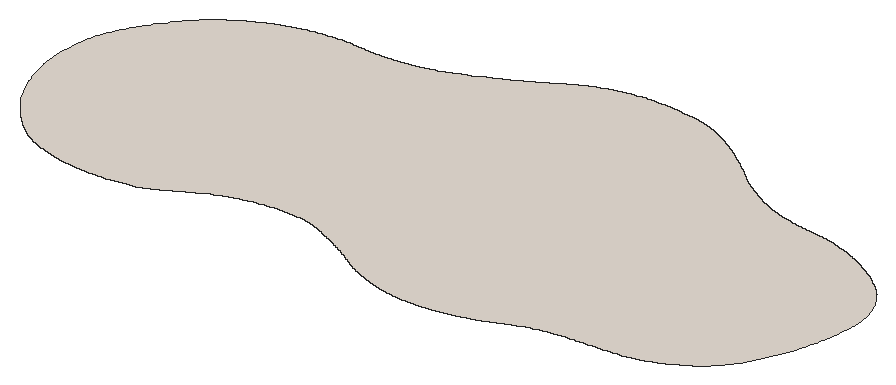
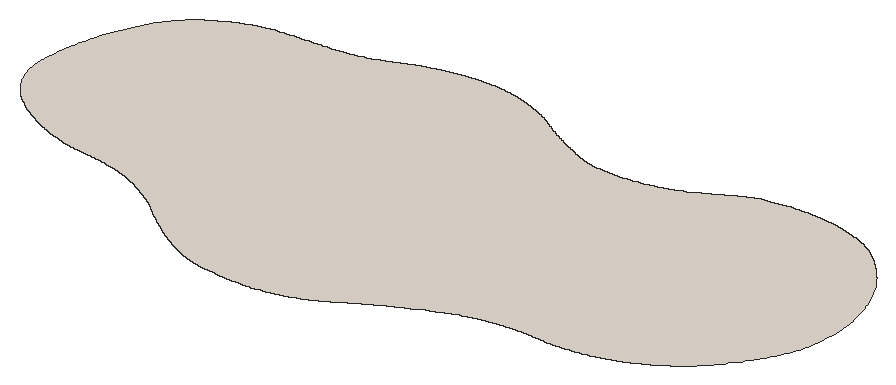
# SketchUp Ruby script. Lengths in inches.
U = 1.inch
M = Sketchup.active_model
def pt(a) = Geom::Point3d.new(a.map { |v| v * U })
def face(e, loops, mat)
  f = e.add_face(loops[0].map { |a| pt(a) })
  loops[1..].each { |l| e.add_face(l.map { |a| pt(a) }).erase! }
  f.material = f.back_material = mat if mat
  f
end
# faces: each face lists its corners as indices into pts; further lists are holes
def faces(e, pts, list, mat = nil) = list.each { |f| face(e, (f[0].is_a?(Array) ? f : [f]).map { |l| l.map { |i| pts[i] } }, mat) }
# xy, xz, yz: faces in a plane at the given z, y or x. An outline is a flat list of corners, or four numbers for a rectangle; further outlines are holes
def ring(l) = l.size == 4 ? [[l[0], l[1]], [l[2], l[1]], [l[2], l[3]], [l[0], l[3]]] : l.each_slice(2).to_a
def flat(e, list, mat, &to3) = list.each { |f| face(e, (f[0].is_a?(Array) ? f : [f]).map { |l| ring(l).map { |u, v| to3.(u, v) } }, mat) }
def xy(e, z, list, mat = nil) = flat(e, list, mat) { |x, y| [x, y, z] }
def xz(e, y, list, mat = nil) = flat(e, list, mat) { |x, z| [x, y, z] }
def yz(e, x, list, mat = nil) = flat(e, list, mat) { |y, z| [x, y, z] }
def lines(e, pts, list) = list.each { |a, b| e.add_line(pt(pts[a]), pt(pts[b])) }
# prism: a flat outline (further loops are holes) pulled along v
def prism(e, loops, v, mat = nil)
  f = face(e, loops, mat); d = Geom::Vector3d.new(v.map { |x| x * U })
  f.pushpull(f.normal.samedirection?(d) ? d.length : -d.length)
end
def box(e, o, s, mat = nil) = prism(e, [[o, [o[0] + s[0], o[1], o[2]], [o[0] + s[0], o[1] + s[1], o[2]], [o[0], o[1] + s[1], o[2]]]], [0, 0, s[2]], mat)
def at(x, y, z, deg = 0) = Geom::Transformation.translation(pt([x, y, z])) * Geom::Transformation.rotation(ORIGIN, Z_AXIS, deg.degrees)
def axes(o, x, y, z) = Geom::Transformation.new([*x, 0, *y, 0, *z, 0, *pt(o).to_a, 1])
def part(name) = M.definitions.add(name)
# library, detail: a bought-in or finely detailed component or shape, given as its bounding box
def library(name, o, s) = part(name).tap { |d| box(d.entities, o, s) }
def detail(e, o, s) = box(e.add_group.entities, o, s)
def put(e, d, t, mat = nil) = e.add_instance(d, t).tap { |i| i.material = mat if mat }
def group(e, t, mat = nil) = e.add_group.tap { |g| g.transformation = t; g.material = mat if mat }.entities
root = M.entities
M.materials.add("Marble_01_1K").color = [230, 221, 211]
xy(root,19,[[347.35,773.18,347.67,773.18,347.88,773.19,347.99,773.19,348.1,773.2,348.2,773.21,348.31,773.21,348.42,773.22,348.52,773.23,348.73,773.25,348.83,773.26,349.01,773.28,349.1,773.3,349.19,773.31,349.43,773.34,349.51,773.36,349.59,773.37,349.66,773.38,349.74,773.4,349.81,773.41,349.89,773.43,349.97,773.44,350.04,773.46,350.12,773.47,350.19,773.49,350.27,773.5,350.34,773.52,350.42,773.54,350.49,773.55,350.57,773.57,350.64,773.59,350.72,773.61,350.79,773.625,350.87,773.64,350.94,773.66,351.02,773.68,351.09,773.7,351.17,773.72,351.24,773.74,351.32,773.76,351.39,773.78,351.46,773.81,351.54,773.83,351.68,773.87,351.76,773.89,351.83,773.92,351.91,773.94,351.98,773.96,352.05,773.99,352.125,774.01,352.2,774.04,352.27,774.0625,352.34,774.09,352.42,774.11,352.49,774.14,352.5625,774.17,352.63,774.19,352.71,774.22,352.78,774.25,352.85,774.27,352.99,774.33,353.07,774.36,353.42,774.51,353.5,774.54,353.64,774.6,353.72,774.63,353.8,774.67,353.96,774.73,354.04,774.77,354.13,774.8,354.21,774.84,354.39,774.91,354.48,774.94,354.57,774.98,354.65,775.01,354.83,775.07,354.92,775.11,355.19,775.2,355.28,775.22,355.55,775.31,355.64,775.33,355.73,775.36,355.82,775.38,355.92,775.41,356.1,775.45,356.19,775.48,356.28,775.5,356.47,775.54,356.65,775.58,356.75,775.59,356.84,775.61,356.94,775.63,357.03,775.65,357.13,775.66,357.35,775.7,357.46,775.71,357.58,775.73,357.71,775.74,357.86,775.76,358.02,775.78,358.2,775.79,358.4,775.81,358.64,775.82,358.9,775.84,359.2,775.84,359.53,775.85,359.87,775.87,360.59,775.93,360.96,775.97,361.31,776.01,361.66,776.06,361.99,776.11,362.3,776.18,362.6,776.24,362.89,776.32,363.16,776.39,363.43,776.48,363.69,776.57,363.95,776.67,364.2,776.77,364.45,776.89,364.7,777,364.94,777.125,365.18,777.26,365.42,777.39,365.65,777.53,366.11,777.83,366.33,777.99,366.55,778.16,366.76,778.33,366.97,778.51,367.17,778.7,367.55,779.1,367.91,779.54,368.23,780,368.39,780.24,368.53,780.49,368.68,780.74,368.82,780.99,369.08,781.51,369.32,782.03,369.43,782.3,369.54,782.5625,369.65,782.83,369.75,783.1,369.93,783.65,370.01,783.93,370.09,784.2,370.17,784.48,370.23,784.76,370.3,785.04,370.36,785.33,370.46,785.89,370.54,786.43,370.57,786.68,370.6,786.91,370.625,787.12,370.64,787.31,370.66,787.47,370.67,787.6,370.68,787.72,370.69,787.8125,370.6875,787.89,370.6875,788.08,370.68,788.14,370.68,788.26,370.67,788.32,370.67,788.38,370.66,788.4375,370.66,788.49,370.65,788.55,370.65,788.61,370.62,788.79,370.61,788.84,370.58,789.02,370.57,789.07,370.56,789.13,370.54,789.1875,370.53,789.25,370.51,789.3,370.5,789.36,370.48,789.42,370.47,789.47,370.45,789.53,370.44,789.59,370.42,789.64,370.4,789.7,370.38,789.75,370.36,789.81,370.34,789.86,370.32,789.92,370.3,789.97,370.28,790.03,370.26,790.08,370.23,790.14,370.21,790.19,370.1875,790.25,370.16,790.3,370.14,790.35,370.11,790.41,370.09,790.46,370.06,790.51,370.03,790.5625,370.01,790.61,369.98,790.67,369.77,791.02,369.73,791.07,369.67,791.17,369.63,791.21,369.57,791.31,369.53,791.36,369.49,791.4,369.46,791.45,369.42,791.49,369.38,791.54,369.35,791.59,369.27,791.67,369.23,791.72,369.19,791.76,369.15,791.81,368.99,791.97,368.95,792.02,368.91,792.06,368.86,792.1,368.78,792.18,368.73,792.21,368.6875,792.25,368.64,792.29,368.6,792.33,368.55,792.37,368.46,792.4375,368.42,792.47,368.375,792.51,368.33,792.54,368.29,792.58,368.17,792.67,368.13,792.69,368.1,792.72,368.07,792.74,368.05,792.76,368.03,792.77,368.01,792.79,367.99,792.8,367.98,792.8125,367.96,792.82,367.95,792.83,367.9375,792.84,367.93,792.85,367.92,792.86,367.9,792.86,367.89,792.875,367.87,792.89,367.78,792.95,367.74,792.98,367.69,793.01,367.64,793.05,367.58,793.08,367.52,793.125,367.45,793.17,367.39,793.21,367.32,793.25,367.25,793.3,367.11,793.38,367.05,793.42,366.42,793.78,366.35,793.8125,366.27,793.85,366.2,793.89,366.13,793.92,366.06,793.96,365.99,793.99,365.91,794.03,365.77,794.09,365.69,794.125,365.62,794.16,365.55,794.19,365.47,794.22,365.33,794.28,365.25,794.3125,365.18,794.34,365.1,794.37,365.03,794.4,364.95,794.43,364.875,794.46,364.8,794.48,364.72,794.51,364.65,794.54,364.57,794.5625,364.5,794.59,364.42,794.61,364.34,794.64,364.27,794.66,364.19,794.68,364.11,794.71,364.04,794.73,363.8,794.79,363.73,794.8125,363.65,794.83,363.41,794.89,363.34,794.91,363.26,794.93,363.18,794.94,363.1,794.96,363.02,794.97,362.94,794.99,362.86,795,362.79,795.02,362.71,795.03,362.63,795.05,362.39,795.08,362.31,795.1,362.15,795.12,362.07,795.125,361.99,795.14,361.91,795.14,361.67,795.17,361.58,795.18,361.5,795.18,361.41,795.19,361.3125,795.2,361.21,795.21,361.11,795.22,360.99,795.23,360.88,795.24,360.76,795.25,360.64,795.27,360.52,795.28,360.39,795.3,360.27,795.3125,360.14,795.33,360.02,795.35,359.89,795.37,359.77,795.39,359.64,795.42,359.52,795.44,359.39,795.47,359.27,795.49,359.15,795.52,359.02,795.55,358.66,795.64,358.54,795.68,358.41,795.71,357.93,795.87,357.8125,795.91,357.69,795.95,357.58,796,357.46,796.04,357.22,796.14,357.11,796.18,356.99,796.23,356.875,796.29,356.76,796.34,356.64,796.39,356.53,796.45,356.42,796.5,356.3,796.56,355.64,796.92,355.53,796.99,355.42,797.05,355.3125,797.12,355.21,797.19,355.1,797.26,355,797.33,354.89,797.4,354.79,797.47,354.69,797.55,354.58,797.62,354.48,797.69,354.38,797.77,354.02,798.05,353.94,798.11,353.87,798.17,353.81,798.22,353.74,798.27,353.68,798.32,353.63,798.37,353.57,798.41,353.52,798.45,353.47,798.5,353.32,798.62,353.26,798.66,353.06,798.82,353,798.86,352.9,798.94,352.84,798.98,352.79,799.02,352.74,799.0625,352.68,799.1,352.58,799.18,352.52,799.22,352.42,799.3,352.36,799.34,352.31,799.375,352.25,799.41,352.15,799.49,352.09,799.52,352.04,799.5625,351.98,799.6,351.93,799.64,351.87,799.67,351.82,799.71,351.76,799.75,351.71,799.78,351.65,799.82,351.59,799.85,351.54,799.89,351.48,799.93,351.43,799.96,351.37,800,351.31,800.03,351.26,800.07,351.2,800.1,351.15,800.14,351.09,800.17,351.03,800.21,350.98,800.24,350.92,800.27,350.86,800.31,350.8,800.34,350.75,800.375,350.69,800.41,350.63,800.44,350.58,800.47,350.52,800.51,350.34,800.6,350.29,800.63,350.23,800.67,350.17,800.7,350.12,800.73,350.07,800.75,350.02,800.78,349.97,800.8,349.93,800.83,349.85,800.87,349.8125,800.89,349.78,800.91,349.74,800.92,349.71,800.9375,349.68,800.95,349.64,800.97,349.61,800.99,349.58,801,349.55,801.02,349.51,801.03,349.48,801.05,349.45,801.0625,349.41,801.08,349.38,801.09,349.35,801.11,349.3125,801.12,349.28,801.14,349.25,801.15,349.21,801.16,349.18,801.18,349.15,801.19,349.11,801.2,349.08,801.22,349.04,801.23,349.01,801.24,348.98,801.26,348.94,801.27,348.91,801.28,348.875,801.3,348.84,801.31,348.81,801.32,348.77,801.33,348.74,801.34,348.7,801.36,348.67,801.37,348.63,801.38,348.6,801.39,348.56,801.4,348.5,801.42,348.46,801.44,348.43,801.45,348.39,801.46,348.36,801.47,348.32,801.48,348.29,801.49,348.25,801.5,348.22,801.51,348.18,801.52,348.15,801.53,348.11,801.54,348.08,801.55,348.04,801.55,348.01,801.5625,347.97,801.57,347.94,801.58,347.86,801.6,347.83,801.61,347.79,801.61,347.76,801.62,347.72,801.63,347.6875,801.64,347.65,801.65,347.62,801.65,347.54,801.67,347.51,801.67,347.47,801.68,347.4375,801.6875,347.4,801.69,347.37,801.7,347.33,801.71,347.29,801.71,347.26,801.72,347.22,801.72,347.1875,801.73,347.15,801.74,347.11,801.74,347.08,801.75,347.04,801.75,347.01,801.76,346.97,801.76,346.93,801.77,346.86,801.77,346.2,801.84,346.0625,801.85,345.91,801.86,345.59,801.88,345.23,801.9,345.04,801.91,344.85,801.91,344.66,801.92,344.1,801.92,343.93,801.91,343.77,801.91,343.61,801.9,343.47,801.89,343.21,801.86,343.09,801.84,342.97,801.83,342.85,801.81,342.74,801.79,342.51,801.75,342.4,801.72,342.29,801.7,342.17,801.68,342.0625,801.65,341.95,801.63,341.84,801.6,341.72,801.57,341.61,801.55,341.51,801.52,341.4,801.49,341.3,801.47,341.21,801.44,341.125,801.42,341.05,801.4,340.98,801.38,340.92,801.36,340.83,801.34,340.79,801.32,340.75,801.3125,340.72,801.3,340.6875,801.29,340.66,801.28,340.59,801.26,340.5625,801.25,340.53,801.24,340.44,801.21,340.4,801.19,340.25,801.14,340.22,801.125,340.18,801.11,340.09,801.08,340.06,801.0625,340.02,801.05,339.99,801.04,339.95,801.02,339.92,801.01,339.83,800.97,339.79,800.95,339.73,800.93,339.61,800.87,339.53,800.84,339.45,800.8,339.36,800.76,339.29,800.72,339.22,800.6875,339.16,800.66,339.11,800.63,338.95,800.55,338.89,800.51,338.85,800.49,338.82,800.48,338.76,800.44,338.73,800.43,338.71,800.41,338.68,800.39,338.62,800.36,338.59,800.34,338.5625,800.32,338.53,800.31,338.5,800.29,338.48,800.27,338.45,800.25,338.42,800.24,338.33,800.18,338.31,800.17,338.22,800.11,338.18,800.09,338.14,800.0625,338.1,800.03,338.04,800,337.97,799.96,337.89,799.91,337.8,799.85,337.6875,799.79,337.57,799.72,337.44,799.64,337.16,799.48,336.86,799.3,336.71,799.22,336.5625,799.13,336.41,799.05,336.25,798.96,336.09,798.875,335.92,798.78,335.74,798.69,335.36,798.49,335.14,798.38,334.91,798.27,334.64,798.14,334.34,797.99,334,797.83,333.61,797.65,333.17,797.45,332.96,797.34,332.76,797.25,332.59,797.17,332.44,797.1,332.31,797.04,332.1875,796.99,332.08,796.95,331.98,796.9,331.88,796.87,331.7,796.79,331.61,796.76,331.53,796.73,331.44,796.7,331.2,796.61,331.12,796.59,331.04,796.56,330.95,796.53,330.875,796.51,330.79,796.48,330.71,796.46,330.625,796.43,330.54,796.41,330.46,796.39,330.38,796.36,330.3,796.34,330.21,796.32,330.05,796.28,329.96,796.26,329.8,796.22,329.71,796.2,329.63,796.18,329.54,796.17,329.46,796.15,329.375,796.13,329.29,796.12,329.21,796.1,329.12,796.09,329.04,796.07,328.95,796.06,328.87,796.05,328.78,796.03,328.7,796.02,328.61,796.01,328.53,796,328.44,795.99,328.36,795.98,328.27,795.97,328.1875,795.96,328.1,795.95,328.02,795.94,327.93,795.9375,327.84,795.93,327.76,795.92,327.67,795.92,327.59,795.91,327.5,795.91,327.42,795.9,327.24,795.9,327.16,795.89,326.39,795.89,326.3,795.9,326.13,795.9,326.04,795.91,325.96,795.91,325.87,795.92,325.79,795.92,325.7,795.93,325.61,795.9375,325.52,795.94,325.42,795.95,325.19,795.95,325.07,795.96,324.93,795.96,324.79,795.95,324.63,795.95,324.47,795.94,324.3,795.94,324.13,795.92,323.79,795.9,323.61,795.88,323.4375,795.86,323.26,795.84,323.09,795.82,322.92,795.79,322.74,795.76,322.4,795.7,322.23,795.66,322.05,795.625,321.88,795.58,321.54,795.5,321.21,795.4,320.87,795.3,320.7,795.24,320.54,795.18,320.375,795.125,320.21,795.0625,320.05,795,319.88,794.93,319.72,794.86,319.5625,794.79,319.4,794.72,319.24,794.64,319.09,794.57,318.77,794.41,318.62,794.32,318.47,794.24,318.3125,794.15,318.16,794.0625,318.01,793.97,317.86,793.88,317.72,793.78,317.57,793.6875,317.43,793.59,317.28,793.49,317.14,793.38,317,793.28,316.86,793.17,316.72,793.0625,316.59,792.95,316.45,792.84,316.32,792.73,316.19,792.61,316.05,792.5,315.93,792.375,315.8,792.26,315.55,792.01,315.43,791.88,315.31,791.76,315.1875,791.63,315.07,791.5,314.95,791.37,314.84,791.23,314.73,791.1,314.4,790.68,314.3,790.54,314.19,790.4,314.09,790.26,313.89,789.96,313.79,789.8,313.68,789.64,313.58,789.46,313.36,789.1,313.25,788.9,313.13,788.7,313.02,788.5,312.92,788.3,312.8125,788.1,312.72,787.9,312.63,787.71,312.55,787.53,312.49,787.36,312.43,787.2,312.375,787.04,312.33,786.88,312.25,786.58,312.22,786.43,312.1875,786.29,312.16,786.14,312.1,785.84,312.08,785.6875,312.06,785.54,312.04,785.39,312.02,785.23,312.01,785.08,311.99,784.93,311.97,784.63,311.97,784.48,311.96,784.32,311.96,783.87,311.97,783.72,311.97,783.5625,311.98,783.41,312,783.11,312.02,782.96,312.03,782.81,312.07,782.51,312.09,782.35,312.12,782.2,312.14,782.05,312.17,781.91,312.2,781.76,312.24,781.61,312.27,781.46,312.31,781.3125,312.35,781.16,312.39,781.01,312.4375,780.85,312.49,780.6875,312.55,780.52,312.61,780.35,312.68,780.16,312.75,779.96,312.84,779.75,312.95,779.51,313.07,779.25,313.39,778.61,313.59,778.23,313.84,777.88,314.0625,777.58,314.26,777.3125,314.45,777.08,314.61,776.88,314.76,776.71,314.91,776.55,315.04,776.41,315.17,776.28,315.29,776.15,315.42,776.03,315.54,775.92,315.65,775.8125,315.77,775.71,315.89,775.61,316,775.51,316.12,775.41,316.36,775.23,316.49,775.14,316.61,775.05,316.74,774.96,317,774.8,317.28,774.64,317.43,774.57,317.59,774.49,317.76,774.42,317.94,774.35,318.14,774.27,318.36,774.2,318.6,774.125,318.86,774.05,319.13,773.98,319.42,773.91,319.72,773.84,320.34,773.72,321.3,773.6,321.62,773.58,322.26,773.56,322.58,773.56,322.91,773.57,323.23,773.59,323.55,773.62,323.86,773.65,324.17,773.6875,324.47,773.73,324.76,773.78,325.02,773.83,325.27,773.88,325.5,773.93,325.69,773.98,325.87,774.02,326.03,774.07,326.18,774.12,326.32,774.17,326.45,774.23,326.59,774.29,326.74,774.36,326.89,774.44,327.23,774.62,327.77,774.92,327.95,775.03,328.31,775.23,328.65,775.43,328.99,775.61,329.15,775.7,329.49,775.88,329.65,775.96,329.99,776.12,330.17,776.2,330.51,776.34,330.6875,776.41,330.86,776.47,331.04,776.54,331.22,776.6,331.39,776.65,331.57,776.71,331.75,776.76,331.93,776.8125,332.12,776.86,332.3,776.9,332.48,776.95,332.66,776.98,332.85,777.02,333.03,777.05,333.22,777.08,333.4,777.11,333.59,777.14,333.78,777.16,333.96,777.18,334.15,777.2,334.34,777.21,334.52,777.22,334.9,777.24,335.46,777.24,335.64,777.23,335.82,777.23,336,777.22,336.17,777.21,336.32,777.19,336.46,777.18,336.59,777.17,336.71,777.15,336.8,777.13,336.89,777.12,337.03,777.08,337.09,777.0625,337.15,777.04,337.2,777.02,337.25,777.01,337.31,776.99,337.41,776.95,337.47,776.93,337.57,776.89,337.68,776.85,337.78,776.81,337.84,776.79,337.89,776.76,337.99,776.72,338.05,776.7,338.2,776.64,338.26,776.62,338.31,776.59,338.41,776.55,338.47,776.53,338.52,776.51,338.57,776.48,338.62,776.46,338.67,776.4375,338.73,776.42,338.78,776.39,338.88,776.35,338.93,776.32,338.98,776.3,339.04,776.28,339.09,776.25,339.14,776.23,339.19,776.2,339.29,776.16,339.34,776.13,339.4,776.11,339.45,776.08,339.5,776.06,339.55,776.03,339.6,776.01,339.65,775.98,339.7,775.96,339.75,775.93,339.8,775.91,339.85,775.88,339.9,775.86,340,775.8,340.05,775.78,340.1,775.75,340.16,775.73,340.26,775.67,340.31,775.65,340.41,775.59,340.45,775.57,340.6,775.48,340.65,775.46,340.85,775.34,340.9,775.32,341.15,775.17,341.19,775.14,341.24,775.12,341.44,775,341.49,774.96,341.61,774.9,341.67,774.86,341.74,774.82,341.8125,774.78,341.89,774.73,341.97,774.68,342.33,774.48,342.43,774.43,342.52,774.38,342.62,774.34,342.71,774.29,342.81,774.24,342.9,774.2,343,774.15,343.3,774.03,343.39,773.99,343.79,773.83,343.89,773.8,343.99,773.76,344.1,773.73,344.2,773.7,344.3,773.66,344.5,773.6,344.61,773.57,344.71,773.55,344.8125,773.52,344.92,773.49,345.02,773.47,345.125,773.45,345.23,773.42,345.33,773.4,345.4375,773.38,345.54,773.36,345.65,773.34,345.75,773.32,345.86,773.31,345.97,773.29,346.07,773.28,346.18,773.26,346.28,773.25,346.5,773.23,346.6,773.22,346.71,773.21,346.82,773.21,346.92,773.2,347.03,773.19,347.14,773.19,347.24,773.1875]],"Marble_01_1K")
